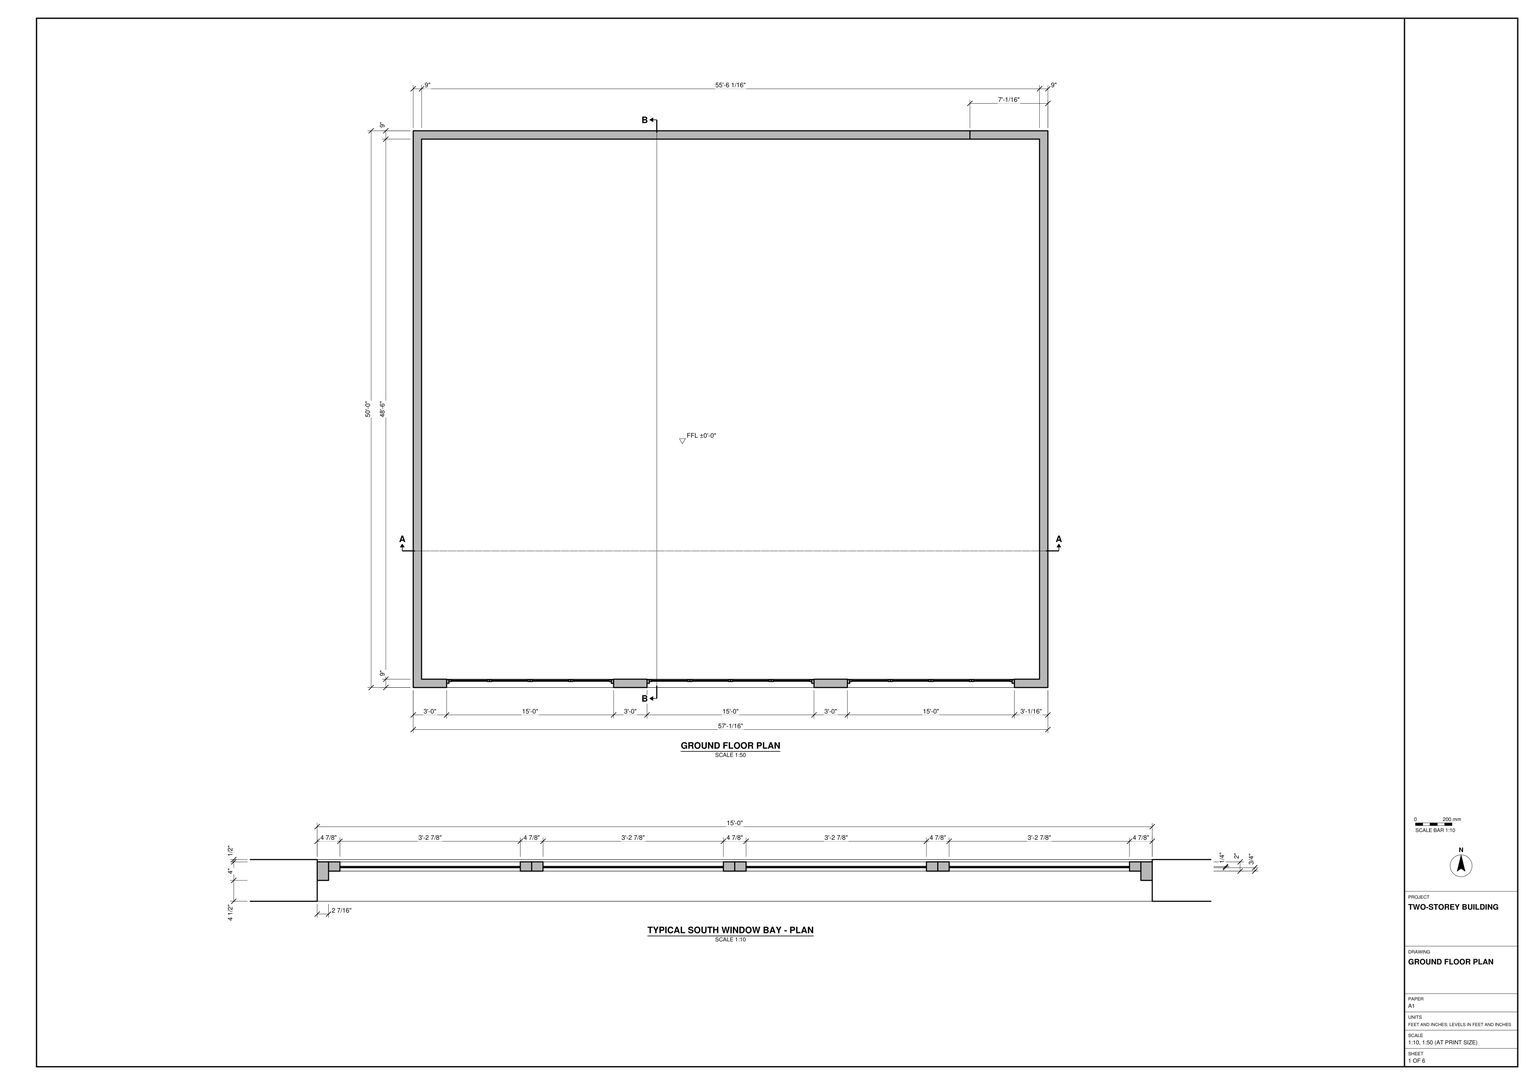
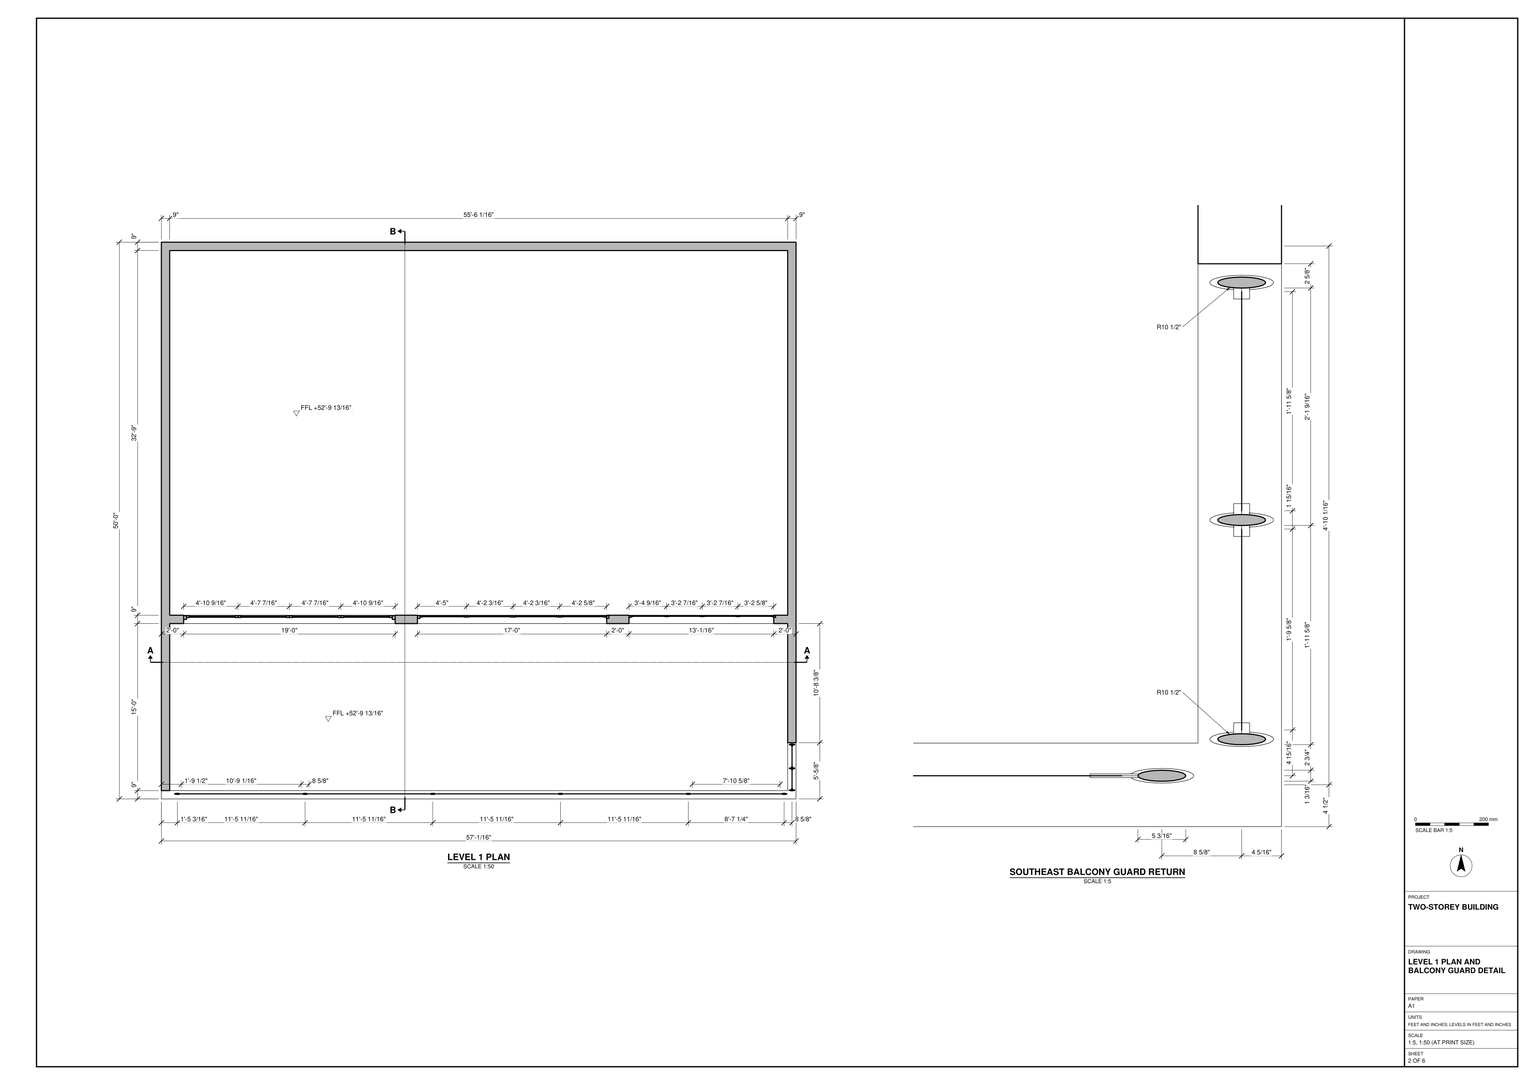
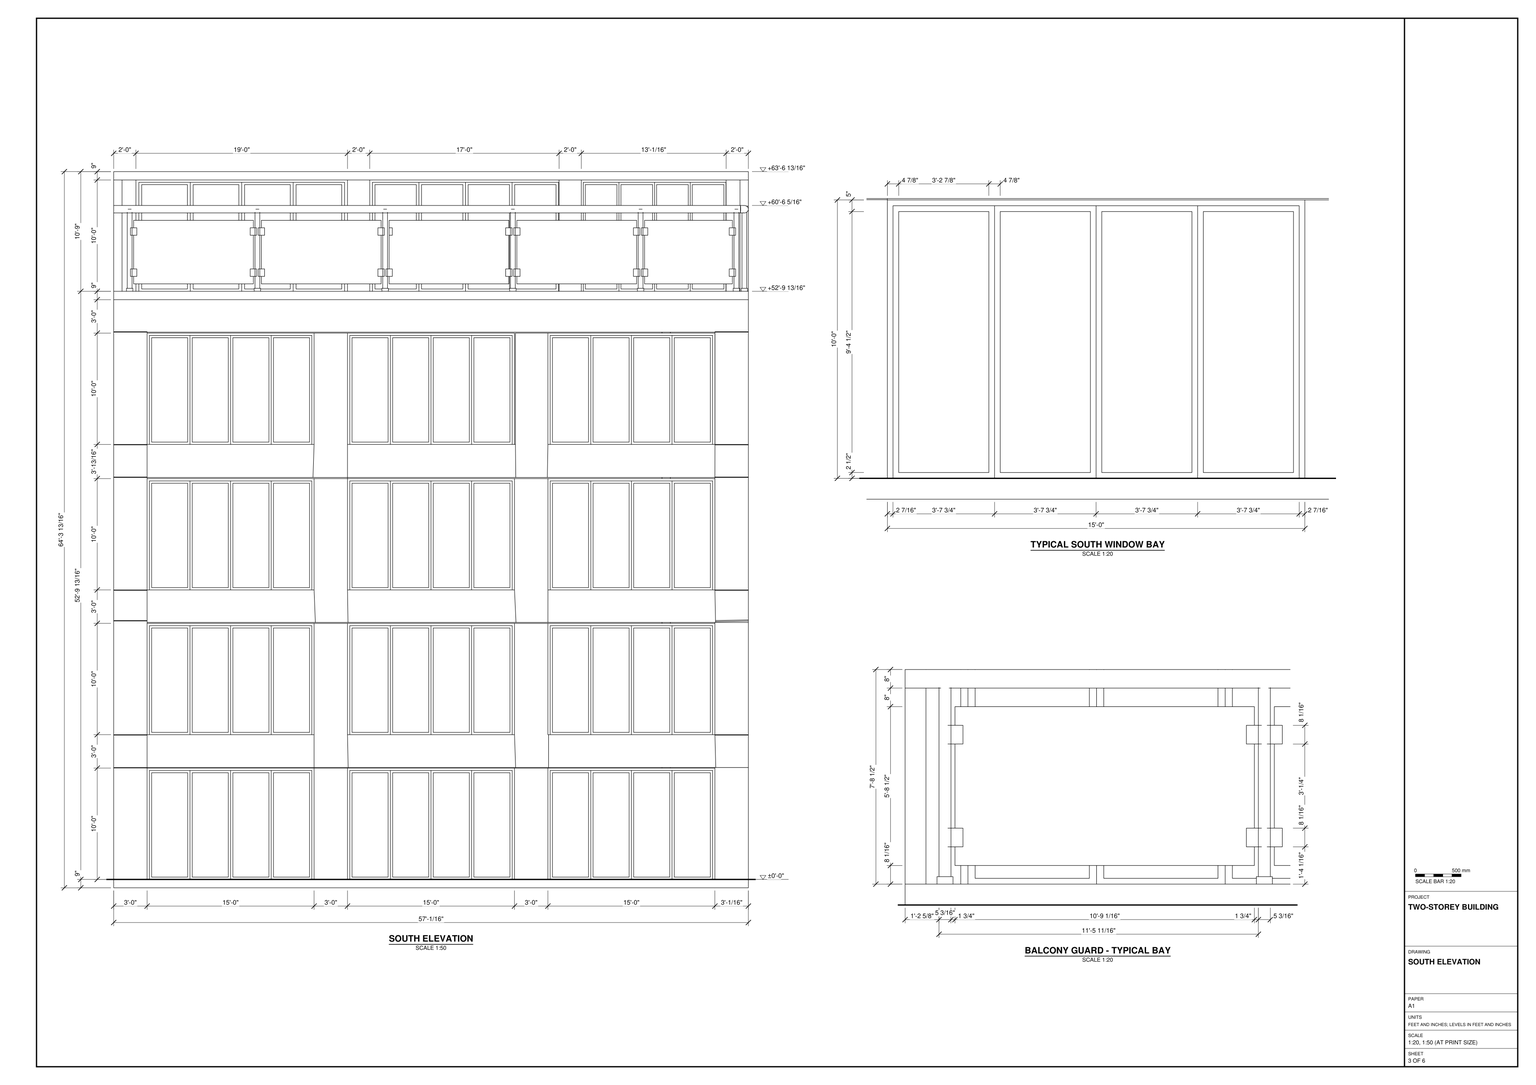
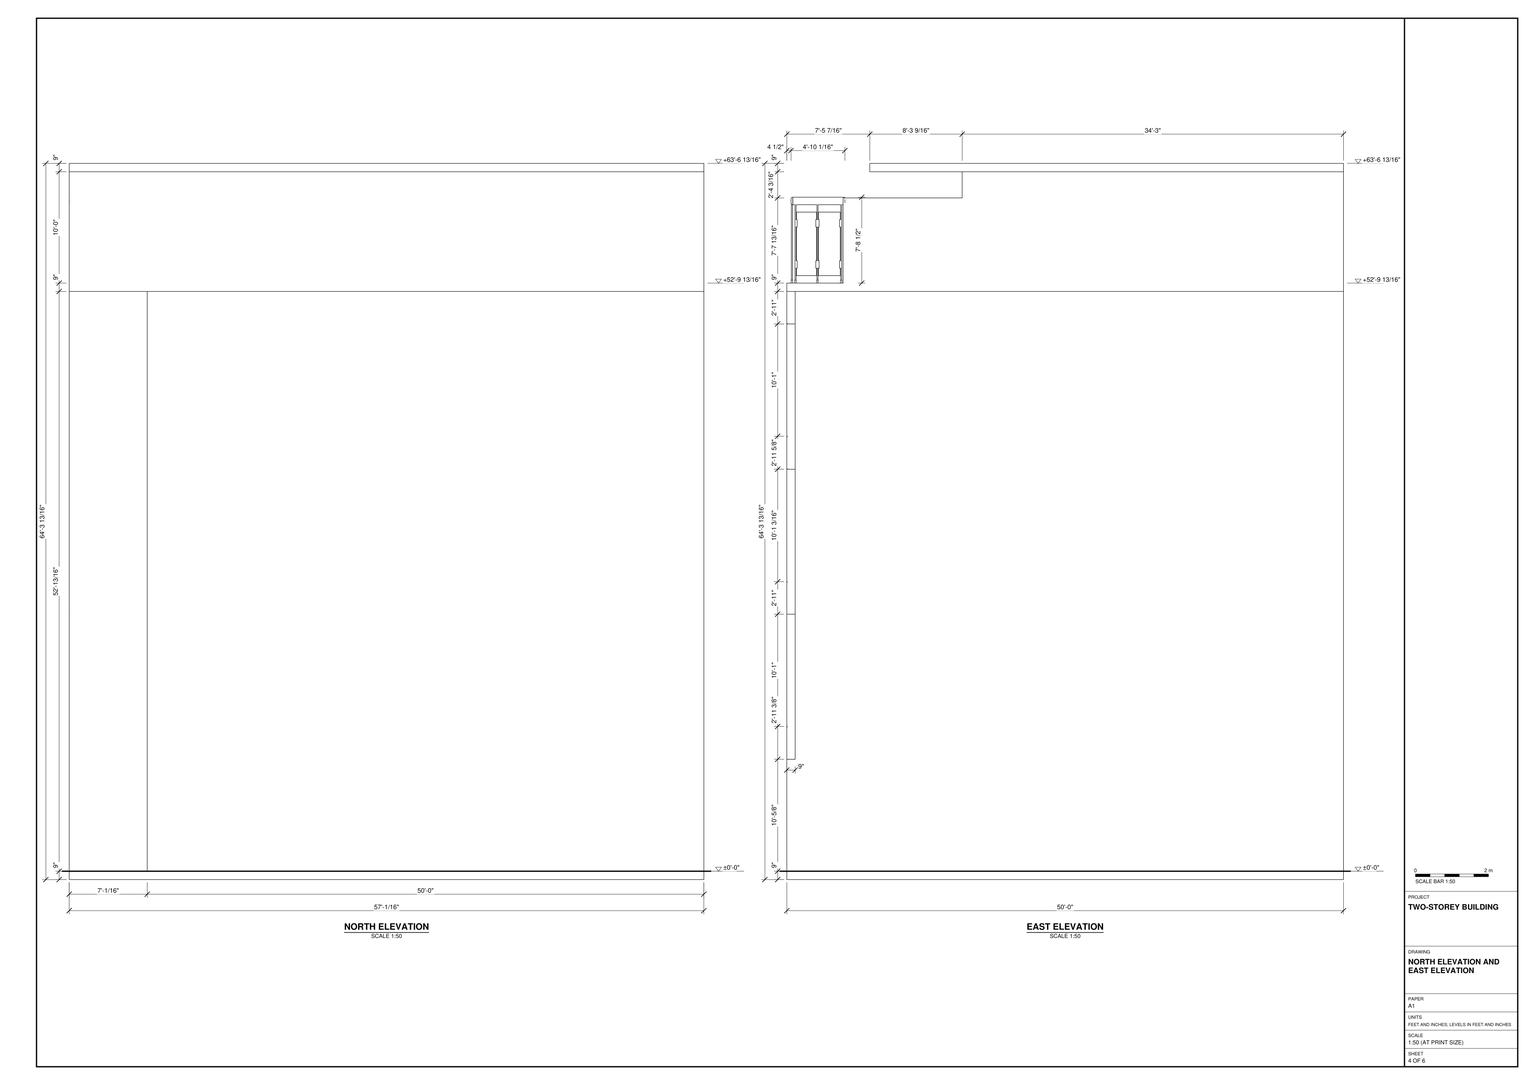
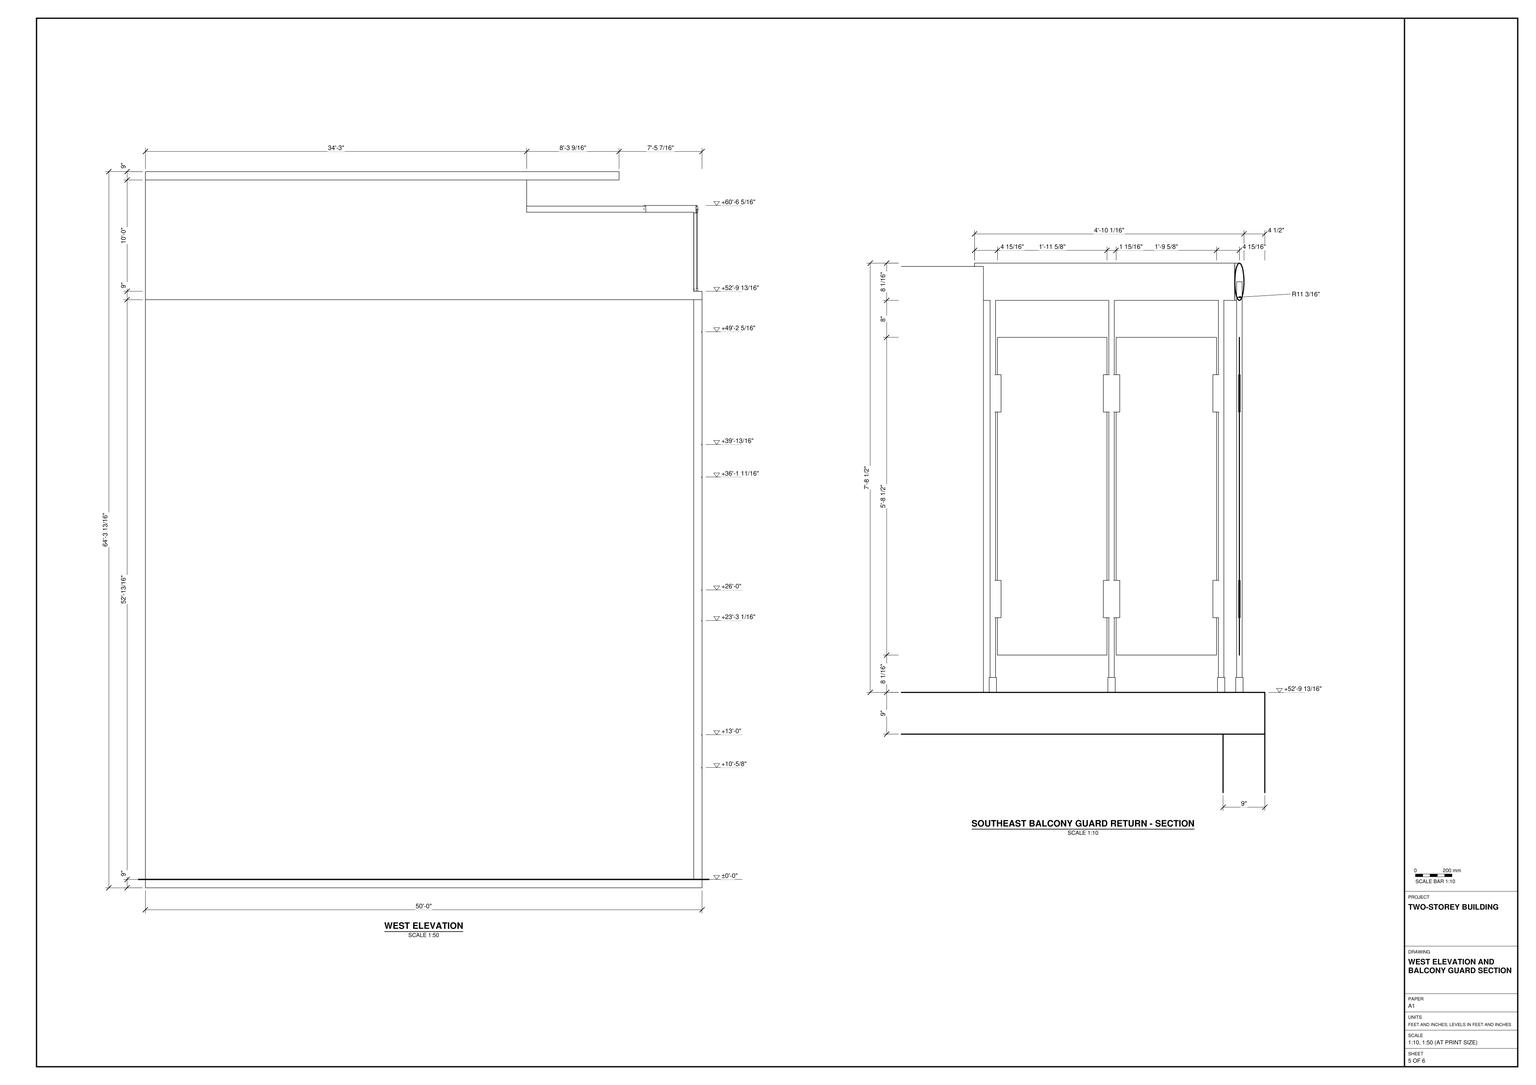
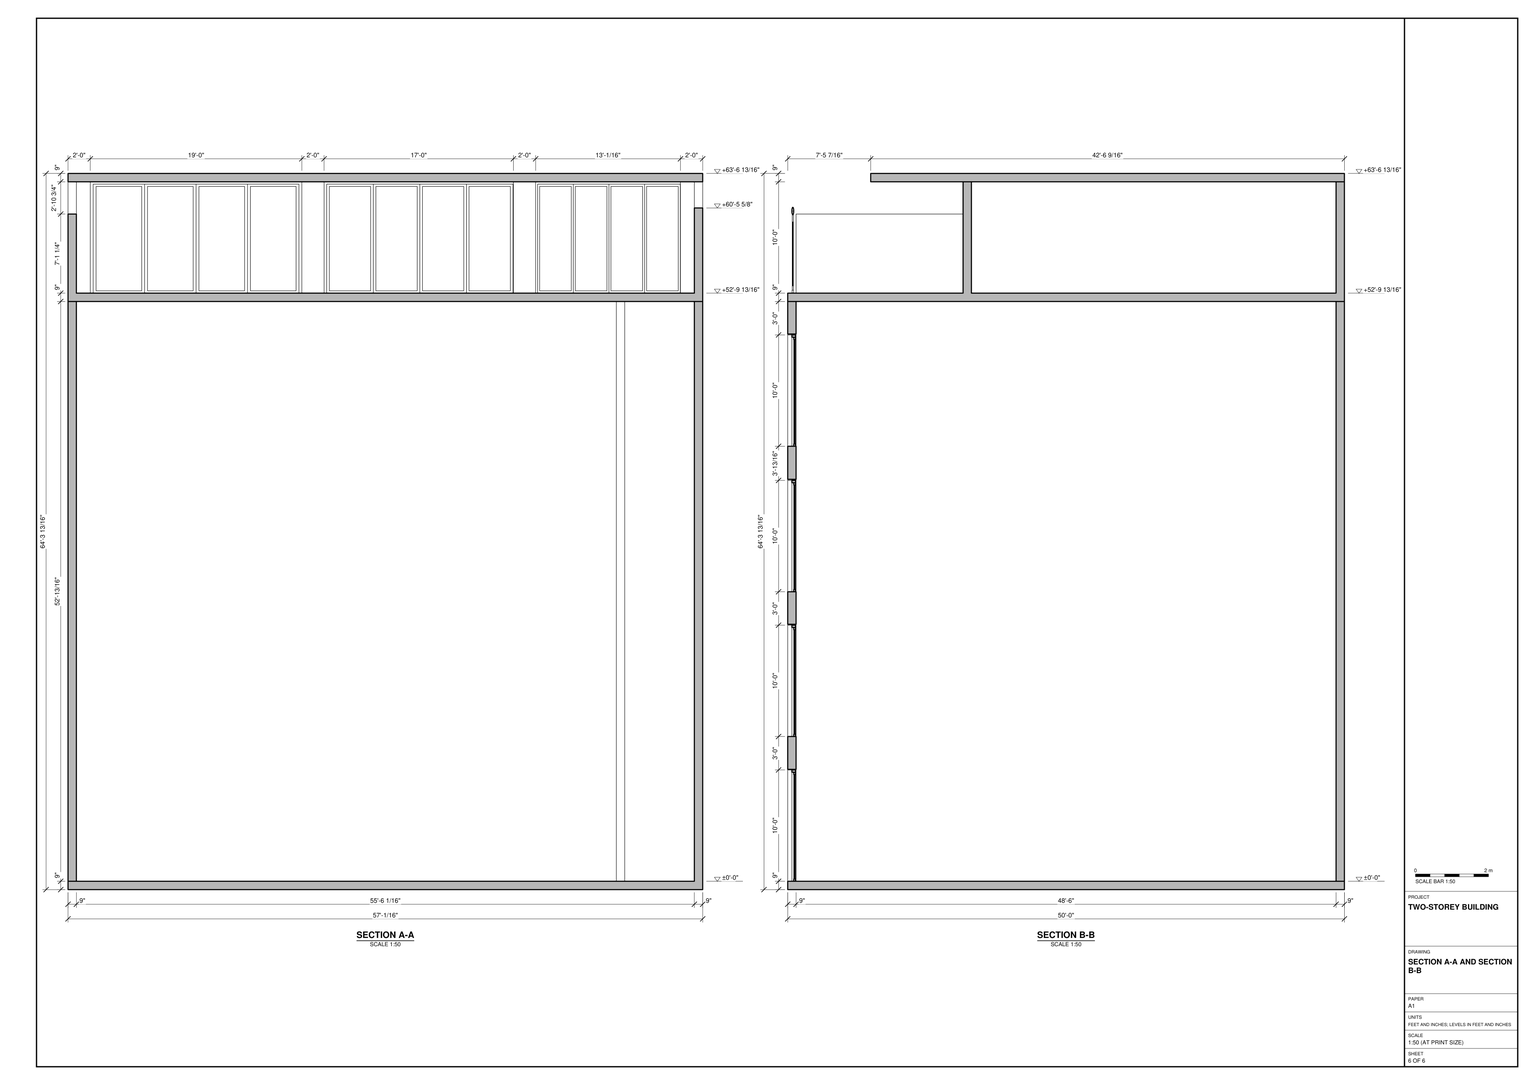
Build the two-storey building in SketchUp from task_files/diagram_01.pdf. Work in feet and inches. The overall size is 57'-1/16" from east to west, 50'-0" from north to south and 64'-3 13/16" from bottom to top. Set the ground floor at ±0'-0" and the upper floor at +52'-9 13/16".

Use the ground floor plan for the rectangular footprint, open interior and 9" perimeter walls. Follow the sections for the floor slabs and roof. On the south face, arrange the lower window bays in three columns and four tiers. Keep the piers aligned and the solid horizontal bands between tiers. Use the typical bay detail to model the frames and the four tall glazed lights within each opening.

Set the upper glazed wall back from the south edge to form the balcony. Follow the upper plan for the unequal glazing bays, the side walls and the guard return at the southeast corner. Model the guard with panels, posts, panel fixings and a continuous top rail.

Keep the walls, slabs, roof and each furniture or joinery piece shown as separate groups or components. Use components for repeated parts. Any decor or loose items shown may be suitable library components. Save one SketchUp model as output_files/two_storey_building_with_stacked_window_bays_and_balcony.skp.

# SketchUp Ruby script. Lengths in inches.
U = 1.inch
M = Sketchup.active_model
def pt(a) = Geom::Point3d.new(a.map { |v| v * U })
def face(e, loops, mat)
  f = e.add_face(loops[0].map { |a| pt(a) })
  loops[1..].each { |l| e.add_face(l.map { |a| pt(a) }).erase! }
  f.material = f.back_material = mat if mat
  f
end
# faces: each face lists its corners as indices into pts; further lists are holes
def faces(e, pts, list, mat = nil) = list.each { |f| face(e, (f[0].is_a?(Array) ? f : [f]).map { |l| l.map { |i| pts[i] } }, mat) }
# xy, xz, yz: faces in a plane at the given z, y or x. An outline is a flat list of corners, or four numbers for a rectangle; further outlines are holes
def ring(l) = l.size == 4 ? [[l[0], l[1]], [l[2], l[1]], [l[2], l[3]], [l[0], l[3]]] : l.each_slice(2).to_a
def flat(e, list, mat, &to3) = list.each { |f| face(e, (f[0].is_a?(Array) ? f : [f]).map { |l| ring(l).map { |u, v| to3.(u, v) } }, mat) }
def xy(e, z, list, mat = nil) = flat(e, list, mat) { |x, y| [x, y, z] }
def xz(e, y, list, mat = nil) = flat(e, list, mat) { |x, z| [x, y, z] }
def yz(e, x, list, mat = nil) = flat(e, list, mat) { |y, z| [x, y, z] }
def lines(e, pts, list) = list.each { |a, b| e.add_line(pt(pts[a]), pt(pts[b])) }
# prism: a flat outline (further loops are holes) pulled along v
def prism(e, loops, v, mat = nil)
  f = face(e, loops, mat); d = Geom::Vector3d.new(v.map { |x| x * U })
  f.pushpull(f.normal.samedirection?(d) ? d.length : -d.length)
end
def box(e, o, s, mat = nil) = prism(e, [[o, [o[0] + s[0], o[1], o[2]], [o[0] + s[0], o[1] + s[1], o[2]], [o[0], o[1] + s[1], o[2]]]], [0, 0, s[2]], mat)
def at(x, y, z, deg = 0) = Geom::Transformation.translation(pt([x, y, z])) * Geom::Transformation.rotation(ORIGIN, Z_AXIS, deg.degrees)
def axes(o, x, y, z) = Geom::Transformation.new([*x, 0, *y, 0, *z, 0, *pt(o).to_a, 1])
def part(name) = M.definitions.add(name)
# library, detail: a bought-in or finely detailed component or shape, given as its bounding box
def library(name, o, s) = part(name).tap { |d| box(d.entities, o, s) }
def detail(e, o, s) = box(e.add_group.entities, o, s)
def put(e, d, t, mat = nil) = e.add_instance(d, t).tap { |i| i.material = mat if mat }
def group(e, t, mat = nil) = e.add_group.tap { |g| g.transformation = t; g.material = mat if mat }.entities
root = M.entities
M.materials.add("[0135_DarkGray]").color = [81, 81, 81]
M.materials.add("[Carrera Marble]").color = [207, 207, 207]
M.materials.add("[Color M07]").color = [58, 58, 58]
M.materials.add("[Formica Beige]").color = [211, 187, 149]
M.materials.add("[Metal Seamed]").color = [118, 119, 115]
M.materials.add("[Translucent Glass Gray]").color = [128, 128, 128]
M.materials["[Translucent Glass Gray]"].alpha = 0.5
c1 = library("korkuluk",[57.56,132.28,15.75],[156.49,58.07,22.63])
c2 = part("dwdwdwdwdw")
g1 = group(c2.entities,at(0,0,0))
prism(g1,[[[0,0,94],[0,35.75,94],[0,35.75,0],[0,0,0]],[[0,33.75,92],[0,2,92],[0,2,2],[0,33.75,2]]],[2,0,0])
g2 = group(c2.entities,at(1,2,2),"[Translucent Glass Gray]")
box(g2,[0,0,0],[0.25,31.75,90])
c3 = part("Group\#31")
p = [[0,145,0],[0,145,94],[0,37.75,0],[0,37.75,94]]
lines(c3.entities,p,[[0,1],[2,0],[1,3],[3,2]])
put(c3.entities,c2,at(0,2,0),"[Color M07]")
put(c3.entities,c2,at(0,37.75,0),"[Color M07]")
put(c3.entities,c2,at(0,73.5,0),"[Color M07]")
put(c3.entities,c2,at(0,109.25,0),"[Color M07]")
g3 = group(c3.entities,at(0,0,0),"[Metal Seamed]")
xy(g3,0,[[0,0,4,2],[0,145,4,147]])
xy(g3,94,[[0,2,4,145]])
xy(g3,96,[[0,0,4,147]])
xz(g3,0,[[0,0,4,96]])
xz(g3,2,[[0,0,4,94]])
xz(g3,145,[[0,0,4,94]])
xz(g3,147,[[0,0,4,96]])
yz(g3,0,[[0,0,0,96,147,96,147,0,145,0,145,94,2,94,2,0]])
yz(g3,4,[[0,0,2,0,2,94,145,94,145,0,147,0,147,96,0,96]])
xy(root,-9,[[0,0,684.0625,600]])
xy(root,0,[[0,0,36,0,36,9,9,9,9,591,600,591,600,600,0,600],[36,0,216,9],[252,0,432,9],[468,0,648,9],[9,9,675.0625,591]])
xy(root,120,[[216,0,252,9],[432,0,468,9]])
xy(root,120.106,[[0,0,36,0.5]])
xy(root,120.606,[[0,0,36,0.5],[36,0,684.0625,9]])
xy(root,120.625,[[648,0,684.0625,9]])
xy(root,155.5,[[0,0,36,0.5],[648.013,0,684.0625,0.5]])
xy(root,156,[[0,0,36,0.5],[36,0,216,9],[252,0,432,9],[468,0,648,9],[648,0,684.0625,0.5]])
xy(root,276,[[216,0,252,9],[432,0,468,9]])
xy(root,276.983,[[36,0,648,9]])
xy(root,278.537,[[0,0,36,0.5]])
xy(root,279.037,[[0,0,36,0.5]])
xy(root,311.5,[[0,0,36,0.5],[648.01,0,684.0625,0.5]])
xy(root,312,[[0,0,36,0.5],[36,0,216,9],[252,0,432,9],[468.031,0,648,9],[648,0,684.0625,0.5]])
xy(root,432,[[216,0,252,9],[432,0,468.031,9]])
xy(root,433.185,[[0,0,36,0.5],[36,0,648,9],[648,0,684.0625,0.5]])
xy(root,433.685,[[0,0,36,0.5],[648.001,0,684.0625,0.5]])
xy(root,468.3125,[[0,0,36,0.5],[648.092,0,684.0625,0.5]])
xy(root,468.8125,[[0,0,36,0.5],[36,0,216,9],[252,0,432.998,9],[468,0,648.092,9],[648.092,0,684.0625,0.5]])
xy(root,588.8125,[[216,0,252,9],[432.998,0,468,9]])
xy(root,589.807,[[0,0,36,0.5],[36,0,648.092,9],[648.092,0,684.0625,0.5]])
xy(root,590.307,[[0,0,36,0.5],[648.092,0,684.0625,0.5]])
xy(root,624.8125,[[0,0,600,9],[600,0,684.0625,9],[0,9,0,600,600,600,600,591,9,591,9,9],[9,9,600,591],[600,9,675.0625,591],
  [675.0625,9,675.0625,591,600,591,600,600,684.0625,600,684.0625,9]])
xy(root,633.8125,[[0,0,684.0625,0,684.0625,60.656,675.0625,60.656,675.0625,9,0,9],[24,189,252,198],[276,189,480,198],[504,189,660.0625,198],[9,198,675.0625,591]])
xy(root,633.8125,[[9,9,675.0625,189]],"[Carrera Marble]")
xy(root,719.044,[[0,9,9,189]])
xy(root,725.625,[[675.0625,60.656,684.0625,189]])
xy(root,753.8125,[[0,89.4375,0,189,24,189,24,198,9,198,9,591,675.0625,591,675.0625,198,660.0625,198,660.0625,189,684.0625,189,684.0625,89.4375],[0,189,24,198],[252,189,276,198],[480,189,504,198],[660.0625,189,684.0625,198],
  [0,198,0,600,684.0625,600,684.0625,198,675.0625,198,675.0625,591,9,591,9,198]])
xy(root,762.8125,[[0,89.4375,684.0625,600]])
xz(root,0,[[648.905,120.606,684.0625,120.606,684.0625,120.625,648.904,120.625],[648.683,276.983,684.0625,276.983,684.0625,278.537,648.666,277.846],[648.666,277.846,684.0625,278.537,684.039,279.727,648.643,279.037],[0,624.8125,684.0625,633.8125]])
xz(root,0,[[36,120.606,216,156],[252.706,120.606,433.209,120.606,432,156,252,156],[468.73,120.606,648,120.606,648,120.625,648.904,120.625,648.013,155.5,648,155.5,648,156,468.73,156],[648,120.606,648.905,120.606,648.904,120.625,648,120.625],[648,155.5,648.013,155.5,648,156],
  [36,276.983,217.355,276.983,216,312,36,312],[252.534,276.983,433.6,276.983,432,312,252,312],[468,276.983,648.683,276.983,648.666,277.846,648.643,279.037,648.01,311.5,648,311.5,648,312,468.031,312],[648,311.5,648.01,311.5,648,312],[36,433.185,214.793,433.185,216,468.8125,36,468.8125],
  [252,433.185,433.368,433.185,432.998,468.8125,252,468.8125],[467.366,433.185,648,433.185,648,433.685,648.001,433.685,648.092,468.8125,468,468.8125],[648,433.185,648.001,433.685,648,433.685]],"[0135_DarkGray]")
xz(root,0,[[0,-9,684.0625,-9,684.0625,120.606,648,120.606,648,0,468,0,468,120,432,120,432,0,252,0,252,120,216,120,216,0,0,0],[0,0,36,120.106],[0,120.606,36,155.5],[216,120.606,252.706,120.606,252,156,252,276,216,276],[433.209,120.606,468.73,120.606,468.73,156,468,156,468,276,432,276,432,156],
  [648.904,120.625,684.0625,120.625,684.0625,155.5,648.013,155.5],[0,156,36,278.537],[648,156,684.0625,276.983],[217.355,276.983,252.534,276.983,252,312,252,432,216,432,216,312],[433.6,276.983,468,276.983,468.031,312,468.031,432,432,432,432,312],
  [684.0625,278.537,684.0625,311.5,648.01,311.5,648.643,279.037,684.039,279.727],[0,279.037,36,311.5],[0,312,36,433.185],[648,312,684.0625,433.185],[214.793,433.185,252,433.185,252,588.8125,216,588.8125,216,468.8125],
  [433.368,433.185,467.366,433.185,468,468.8125,468,588.8125,432.998,588.8125,432.998,468.8125],[0,433.685,36,468.3125],[648.001,433.685,684.0625,433.685,684.0625,468.3125,648.092,468.3125,648.092,468.8125],[0,468.8125,36,589.807],[648.092,468.8125,684.0625,589.807],
  [36,589.807,648.092,589.807,648.092,590.307,684.0625,590.307,684.0625,624.8125,0,624.8125,0,590.307,36,590.307]],"[Formica Beige]")
xz(root,0.5,[[0,120.106,36,120.606],[0,155.5,36,156],[648.013,155.5,684.0625,155.5,684.0625,156,648,156],[0,278.537,36,279.037],[0,311.5,36,312],
  [648.01,311.5,684.0625,311.5,684.0625,312,648,312],[0,433.185,36,433.685],[648,433.185,684.0625,433.185,684.0625,433.685,648.001,433.685],[0,468.3125,36,468.8125],[648.092,468.3125,684.0625,468.8125],
  [0,589.807,36,590.307],[648.092,589.807,684.0625,590.307]])
xz(root,9,[[[9,0,9,624.8125,675.0625,624.8125,675.0625,120.625,648,120.625,648,120.606,36,120.606,36,0],[36,468.8125,216,468.8125,216,588.8125,252,588.8125,252,468.8125,432.998,468.8125,432.998,588.8125,468,588.8125,468,468.8125,648.092,468.8125,648.092,589.807,36,589.807],[36,312,216,312,216,432,252,432,252,312,432,312,432,432,468.031,432,468.031,312,648,312,648,433.185,36,433.185],[36,156,216,156,216,276,252,276,252,156,432,156,432,276,468,276,468,156,648,156,648,276.983,36,276.983]],[216,0,252,120],[432,0,468,120],[648,0,675.0625,120.606],[648,120.606,675.0625,120.625],
  [675.0625,120.606,684.0625,120.625],[675.0625,120.625,684.0625,276.983],[675.0625,276.983,684.0625,433.185],[675.0625,433.185,684.0625,589.807],[675.0625,589.807,684.0625,624.8125],
  [0,633.8125,9,719.044]])
xz(root,60.656,[[675.0625,633.8125,684.0625,725.625]])
xz(root,89.4375,[[0,753.8125,684.0625,762.8125]])
xz(root,189,[[0,719.044,9,753.8125],[675.0625,725.625,684.0625,753.8125]])
xz(root,189,[[9,633.8125,24,753.8125],[252,633.8125,276,753.8125],[480,633.8125,504,753.8125],[660.0625,633.8125,675.0625,753.8125]],"[Formica Beige]")
xz(root,198,[[9,633.8125,24,753.8125],[252,633.8125,276,753.8125],[480,633.8125,504,753.8125],[660.0625,633.8125,675.0625,753.8125]])
xz(root,591,[[9,0,591,624.8125],[591,0,600,624.8125],[600,0,675.0625,624.8125],[9,633.8125,675.0625,753.8125]])
xz(root,600,[[0,-9,0,0,600,0,600,624.8125,684.0625,624.8125,684.0625,-9],[0,0,600,624.8125],[0,624.8125,684.0625,753.8125],[0,753.8125,684.0625,762.8125]])
yz(root,0,[[0,-9,600,0],[0,0,0,120.106,0.5,120.106,0.5,120.606,0,120.606,0,155.5,0.5,155.5,0.5,156,0,156,0,278.537,0.5,278.537,0.5,279.037,0,279.037,0,311.5,0.5,311.5,0.5,312,0,312,0,433.185,0.5,433.185,0.5,433.685,0,433.685,0,468.3125,0.5,468.3125,0.5,468.8125,0,468.8125,0,589.807,0.5,589.807,0.5,590.307,0,590.307,0,624.8125,9,624.8125,9,0],[9,0,600,624.8125],[0,624.8125,0,633.8125,9,633.8125,9,719.044,189,719.044,189,753.8125,600,753.8125,600,624.8125],[89.4375,753.8125,600,762.8125]])
yz(root,9,[[9,0,591,624.8125],[9,633.8125,189,719.044],[198,633.8125,591,753.8125]])
yz(root,24,[[189,633.8125,198,753.8125]])
yz(root,36,[[0,0,9,0,9,120.606,0.5,120.606,0.5,120.106,0,120.106],[0,155.5,0.5,156],[0,156,9,276.983],[0,278.537,0.5,279.037],[0,311.5,0.5,312],
  [0,312,9,433.185],[0,433.185,0.5,433.685],[0,468.3125,0.5,468.8125],[0,468.8125,9,589.807],[0,589.807,0.5,590.307]])
yz(root,216,[[0,0,9,120],[0,156,9,276],[0,312,9,432],[0,468.8125,9,588.8125]])
yz(root,252,[[0,0,9,120],[0,156,9,276],[0,312,9,432],[0,468.8125,9,588.8125],[189,633.8125,198,753.8125]])
yz(root,276,[[189,633.8125,198,753.8125]])
yz(root,432,[[0,0,9,120],[0,156,9,276],[0,312,9,432]])
yz(root,432.998,[[0,468.8125,9,588.8125]])
yz(root,468,[[0,0,9,120],[0,156,9,276],[0,468.8125,9,588.8125]])
yz(root,468.031,[[0,312,9,432]])
yz(root,480,[[189,633.8125,198,753.8125]])
yz(root,504,[[189,633.8125,198,753.8125]])
yz(root,600,[[591,0,600,624.8125]])
yz(root,648,[[0,0,9,120.625],[0,156,9,276.983],[0,312,9,433.185]])
yz(root,648.092,[[0,468.3125,0.5,468.8125],[0,468.8125,9,589.807],[0,589.807,0.5,590.307]])
yz(root,660.0625,[[189,633.8125,198,753.8125]])
yz(root,675.0625,[[9,0,591,624.8125],[60.656,633.8125,189,725.625],[198,633.8125,591,753.8125]])
yz(root,684.0625,[[0,-9,600,-9,600,624.8125,9,624.8125,9,120.606,0,120.606],[0,120.606,9,120.625],[0,120.625,9,120.625,9,276.983,0,276.983,0,156,0.5,156,0.5,155.5,0,155.5],[0,276.983,9,276.983,9,433.185,0,433.185,0,312,0.5,312,0.5,311.5,0,311.5],[0.5,433.185,9,433.185,9,589.807,0,589.807,0,468.8125,0.5,468.8125,0.5,468.3125,0,468.3125,0,433.685,0.5,433.685],
  [0.5,589.807,9,589.807,9,624.8125,0,624.8125,0,590.307,0.5,590.307],[0,624.8125,600,624.8125,600,753.8125,189,753.8125,189,725.625,60.656,725.625,60.656,633.8125,0,633.8125],[89.4375,753.8125,600,762.8125]])
p = [[648,0,156],[648.013,0,155.5],[648.013,0.5,155.5],[648,0.5,156],[648,0,312],[648.01,0,311.5],
  [648.01,0.5,311.5],[648,0.5,312],[648.001,0,433.685],[648,0,433.185],[648,0.5,433.185],[648.001,0.5,433.685],
  [36,4.5,120],[36,0,120],[252,4.5,432],[252,0,468.8125]]
faces(root,p,[[0,1,2,3],[4,5,6,7],[8,9,10,11]])
lines(root,p,[[12,13],[14,15]])
put(root,c1,axes([-251.6,-127.78,569.45],[4.37117,0,0],[0,1,0],[0,0,4.08728]))
put(root,c3,axes([36,8.5,0],[0,-1,0],[1.22449,0,0],[0,0,1.25]))
put(root,c3,axes([252,8.5,0],[0,-1,0],[1.22449,0,0],[0,0,1.25]))
put(root,c3,axes([468,8.5,0],[0,-1,0],[1.22449,0,0],[0,0,1.25]))
put(root,c3,axes([36,8.5,156],[0,-1,0],[1.22449,0,0],[0,0,1.25]))
put(root,c3,axes([252,8.5,156],[0,-1,0],[1.22449,0,0],[0,0,1.25]))
put(root,c3,axes([468,8.5,156],[0,-1,0],[1.22449,0,0],[0,0,1.25]))
put(root,c3,axes([36,8.5,312],[0,-1,0],[1.22449,0,0],[0,0,1.25]))
put(root,c3,axes([252,8.5,312],[0,-1,0],[1.22449,0,0],[0,0,1.25]))
put(root,c3,axes([468.03,8.5,312],[0,-1,0],[1.22449,0,0],[0,0,1.25]))
put(root,c3,axes([36,8.5,468.8125],[0,-1,0],[1.22449,0,0],[0,0,1.25]))
put(root,c3,axes([252,8.5,468.8125],[0,-1,0],[1.22449,0,0],[0,0,1.25]))
put(root,c3,axes([468,8.5,468.8125],[0,-1,0],[1.22449,0,0],[0,0,1.25]))
put(root,c3,axes([24,197.5,633.8125],[0,-1,0],[1.55102,0,0],[0,0,1.25]))
put(root,c3,axes([276,197.5,633.8125],[0,-0.73,0],[1.40398,0,0],[0,0,1.25]))
put(root,c3,axes([504,197.5,633.8125],[0,-0.4818,0],[1.07489,0,0],[0,0,1.25]))
